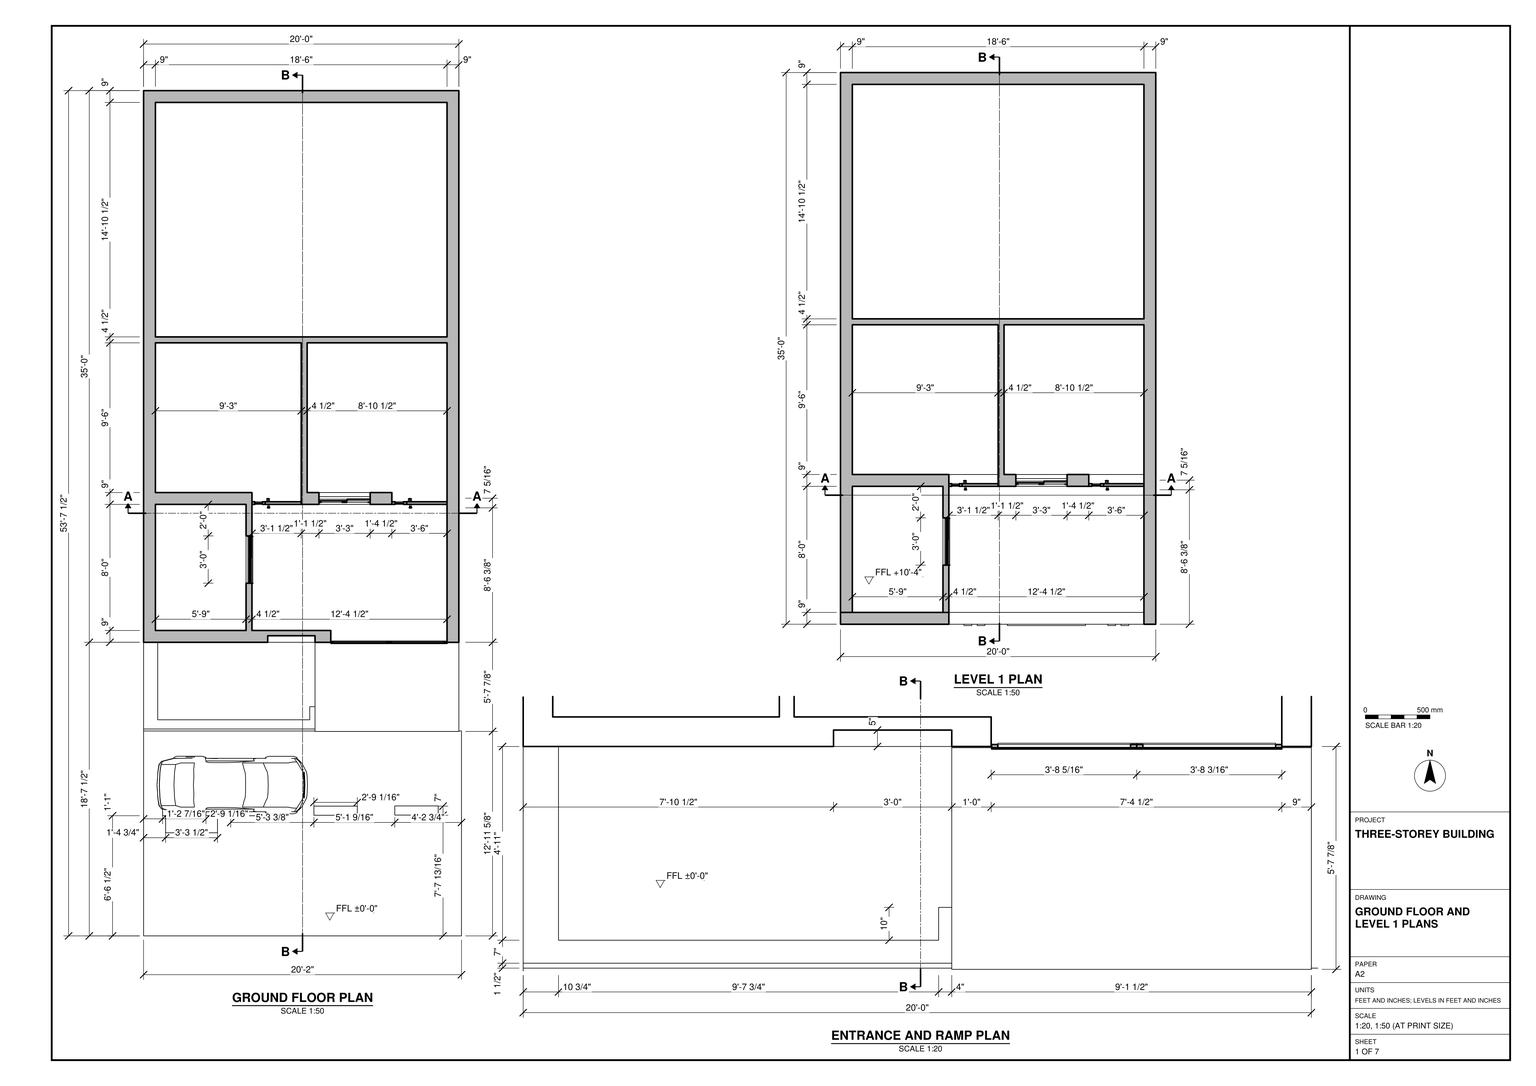
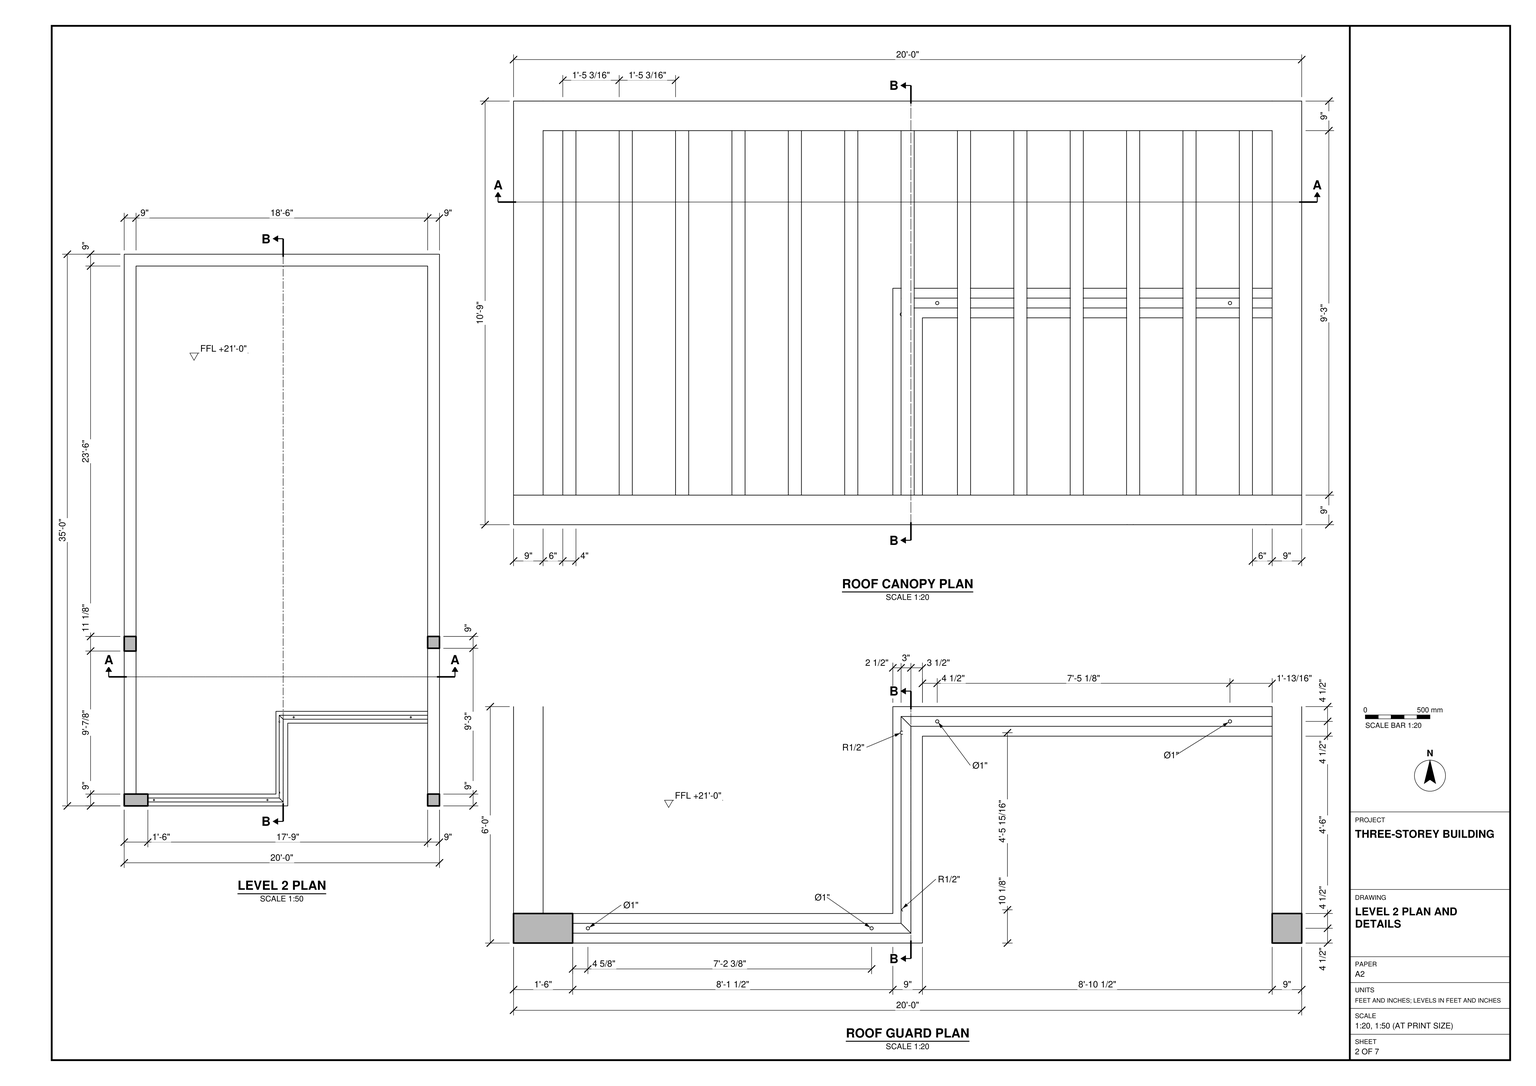
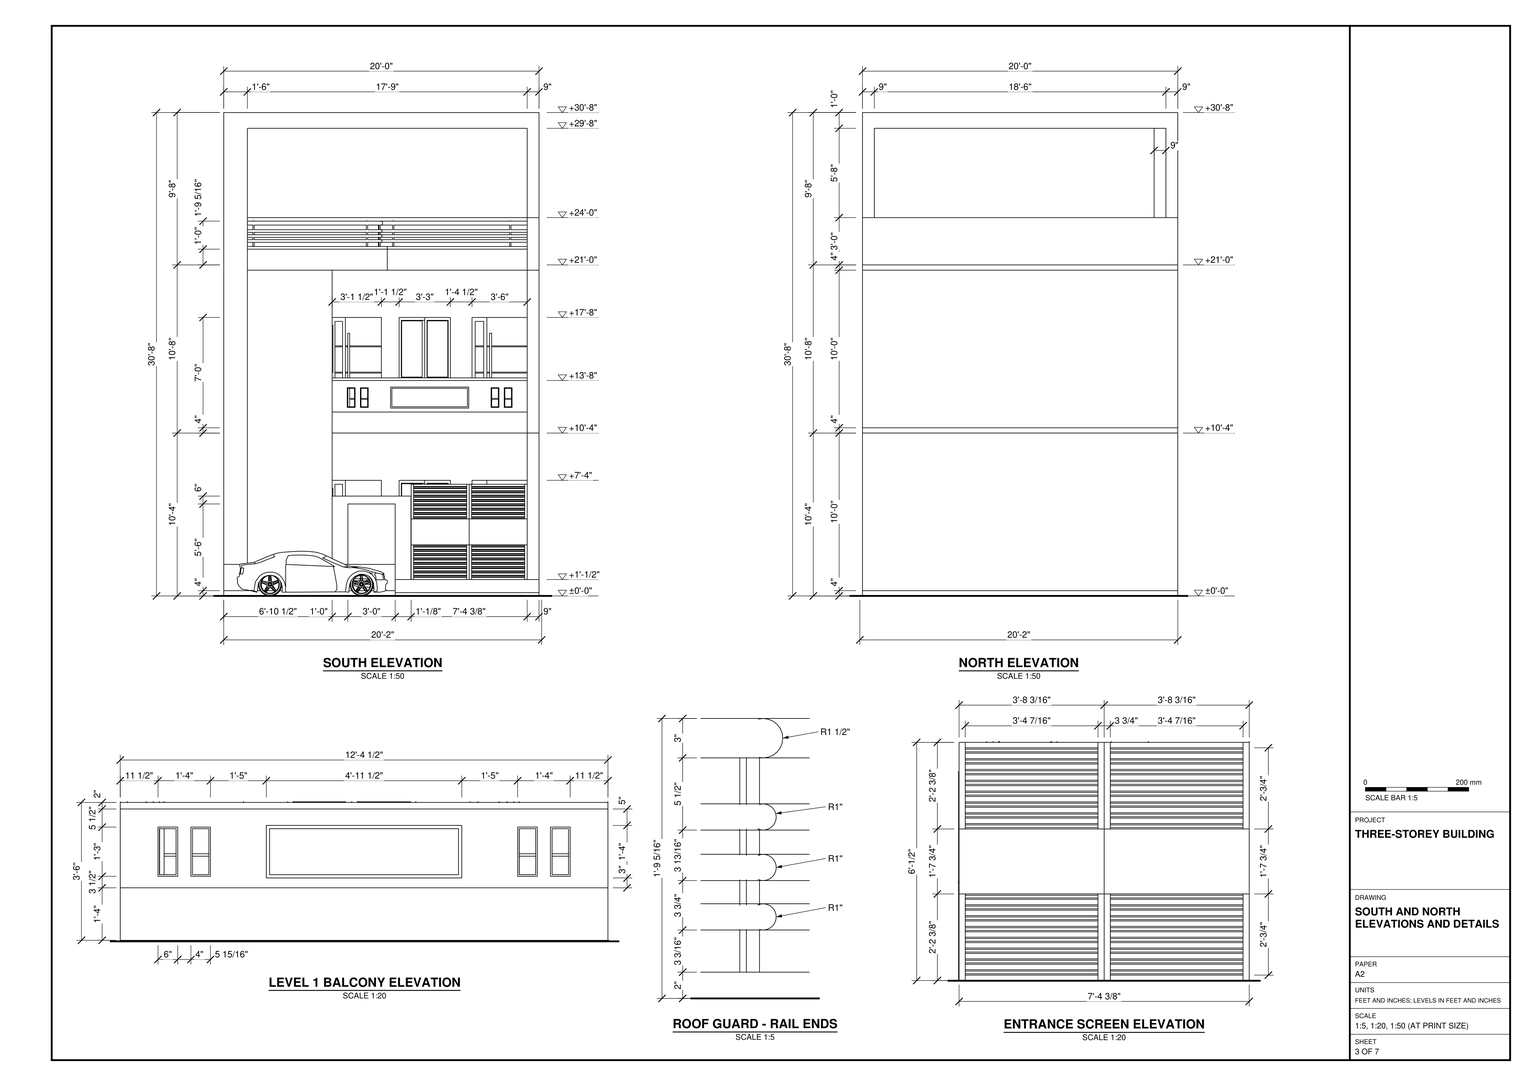
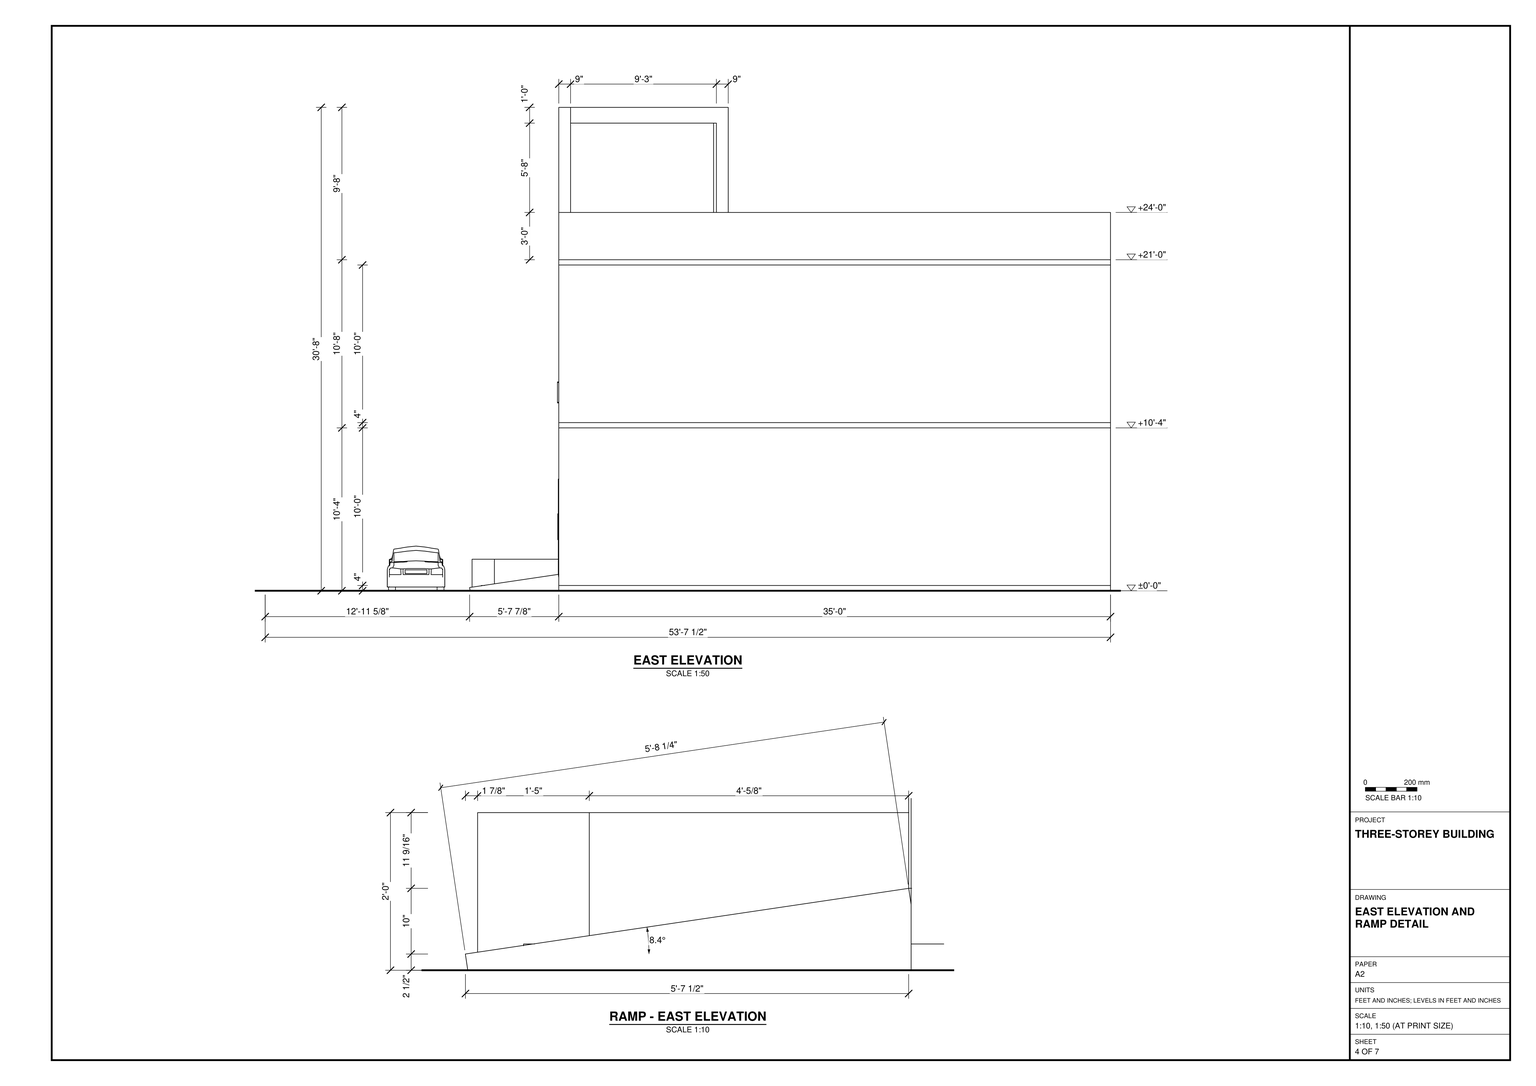
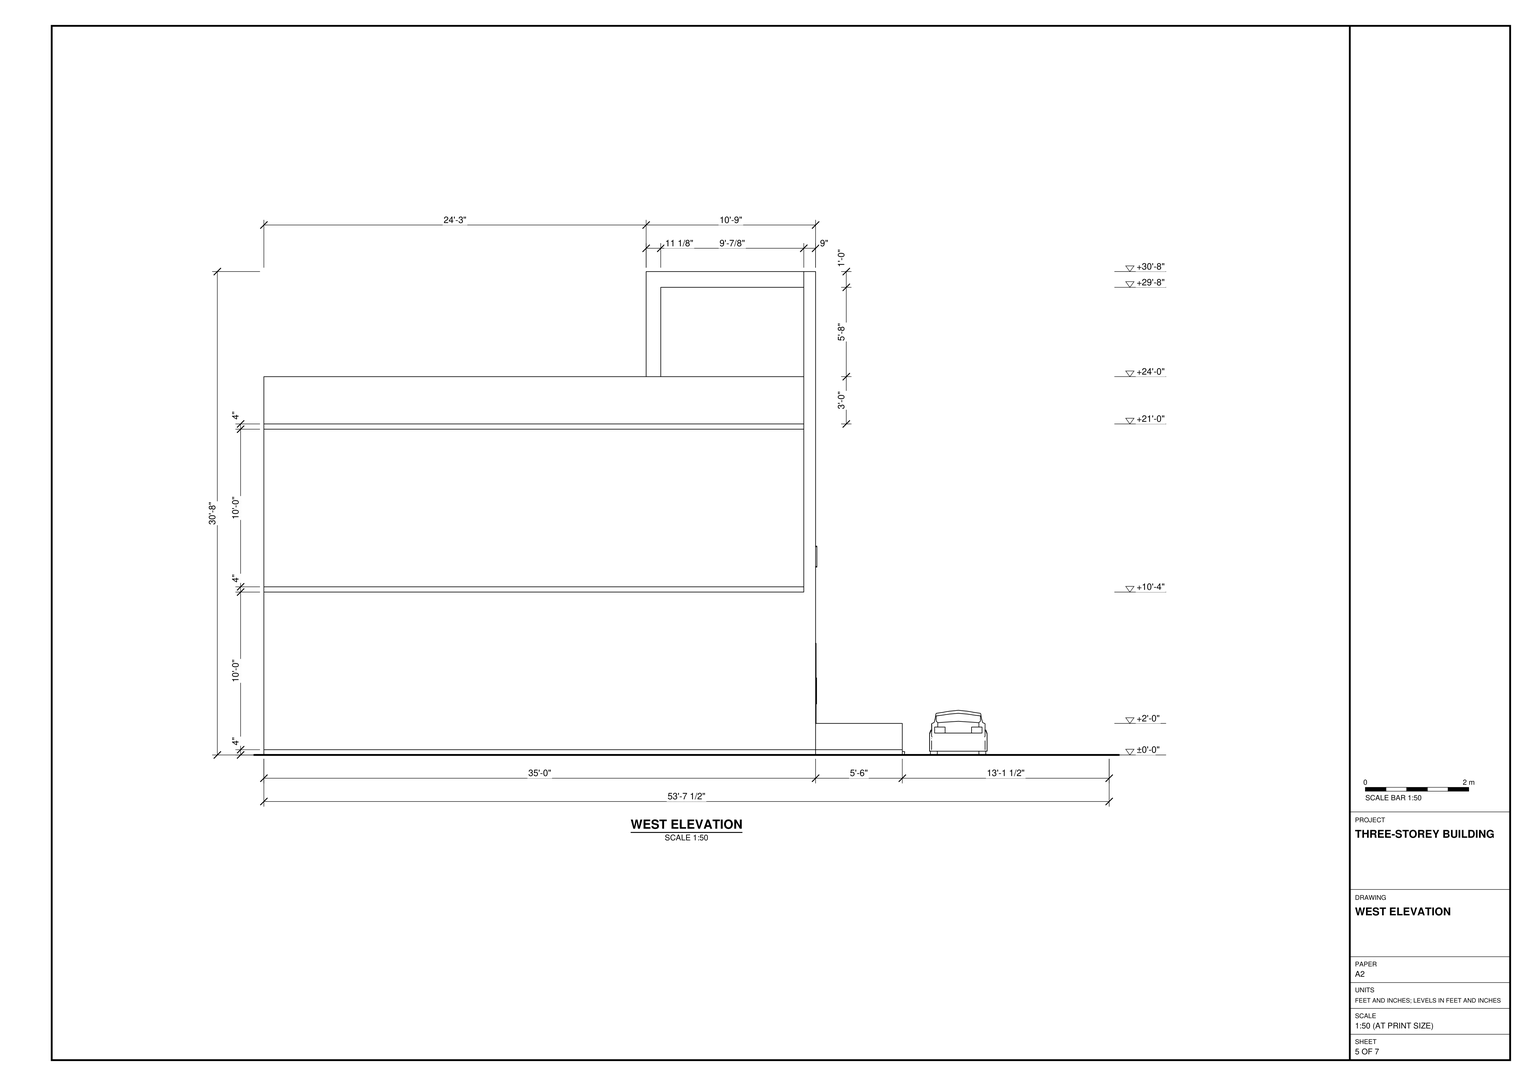
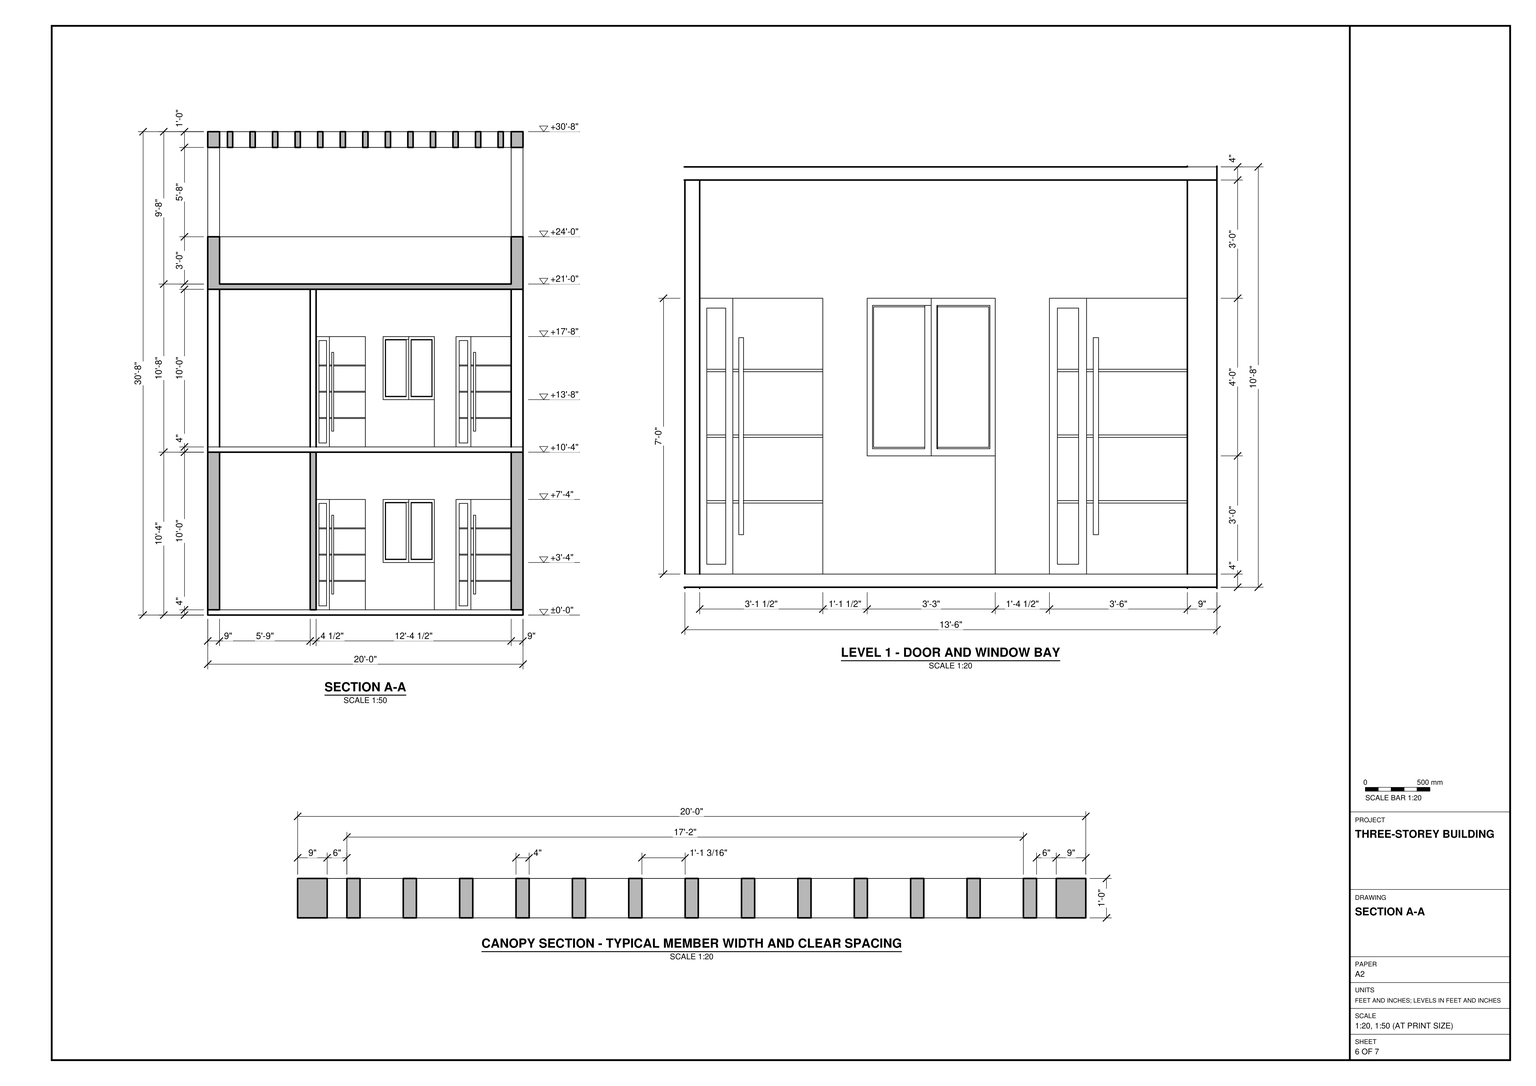
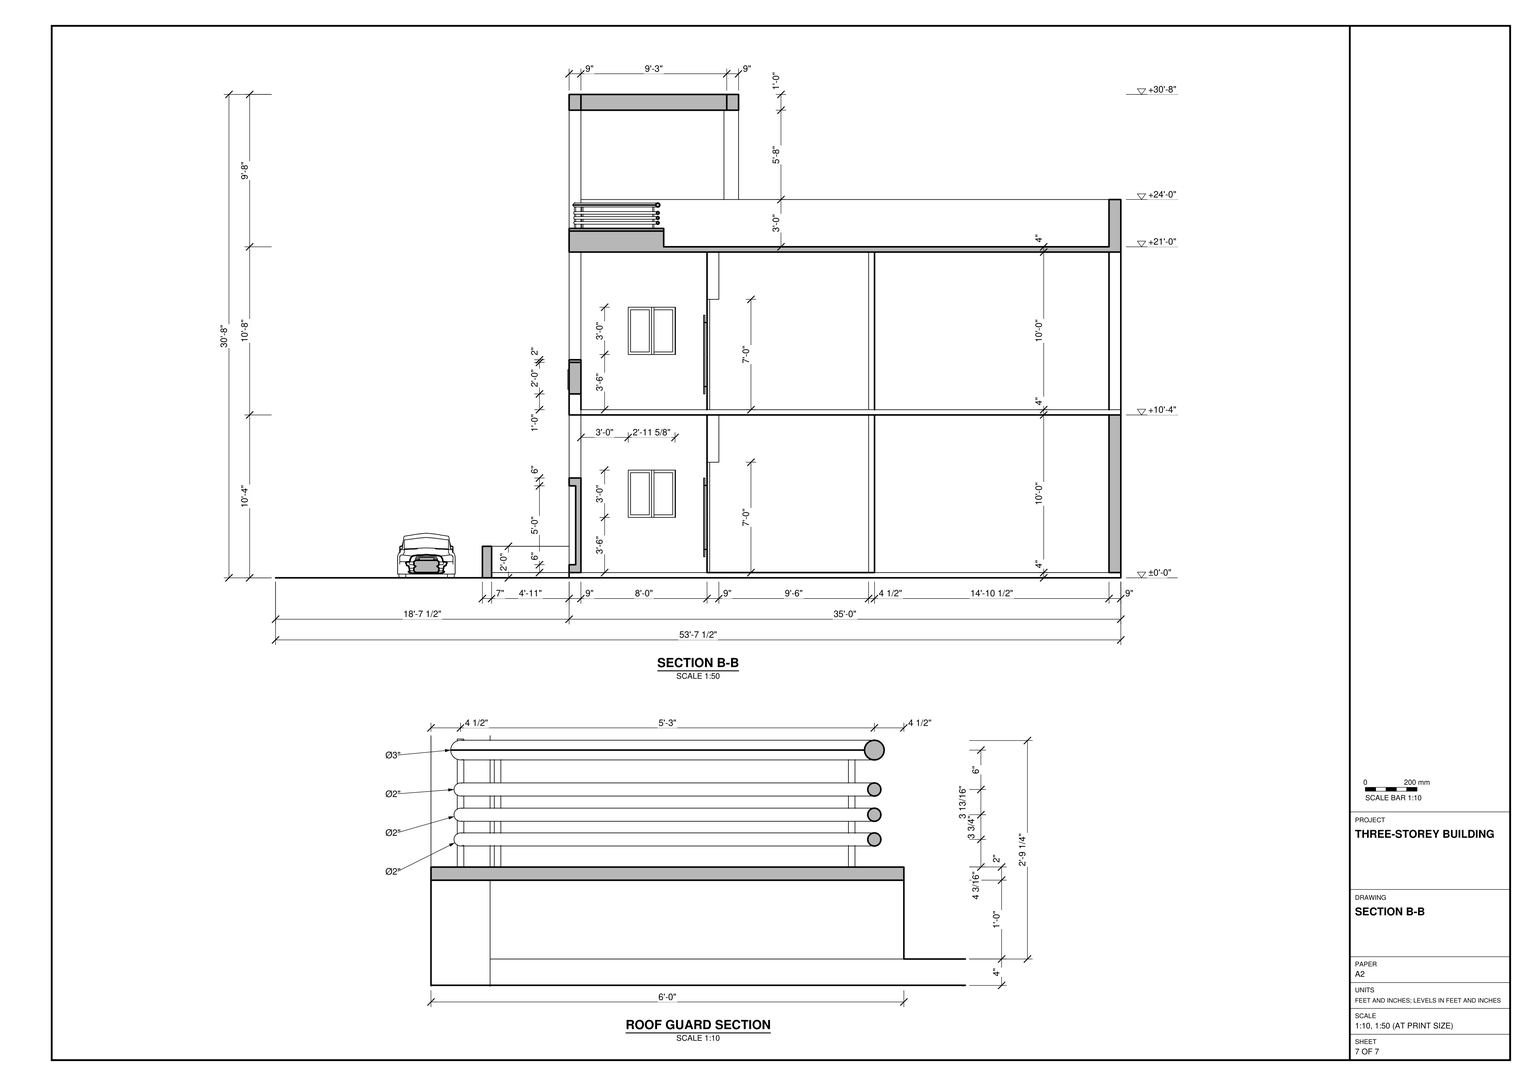
Build the three-storey building and its entrance forecourt in SketchUp from task_files/diagram_01.pdf. Work in feet and inches. The complete model, including the forecourt, is 20'-2" wide, 53'-7 1/2" deep and 30'-8" high. Set the floor levels at ±0'-0", +10'-4" and +21'-0".

Use the 20'-0" by 35'-0" building footprint to lay out the floor slabs and walls. Follow the plans for the 9" perimeter walls, the thinner 4 1/2" partitions and the locations of the door and window openings. On the two lower floors, retain the full-width rear room, the two rooms side by side in the middle and the narrower enclosed space at the front left.

At the south entrance, model the ramp, landing and two-leaf screen. Place the car across the forecourt as shown. Above the entrance, model the recessed openings and the balcony front with its wide central panel and paired narrow panels. At roof level, follow the stepped front edge of the terrace with horizontal guardrails, and build the supported canopy with its parallel overhead members. Decor and loose items, including the car, may be any suitable library components.

Keep walls, slabs, roof elements and each furniture or joinery piece in separate groups or components, and use components for repeated parts. Save one SketchUp model as output_files/three_storey_building_with_roof_terrace_and_ramp.skp.

# SketchUp Ruby script. Lengths in inches.
U = 1.inch
M = Sketchup.active_model
def pt(a) = Geom::Point3d.new(a.map { |v| v * U })
def face(e, loops, mat)
  f = e.add_face(loops[0].map { |a| pt(a) })
  loops[1..].each { |l| e.add_face(l.map { |a| pt(a) }).erase! }
  f.material = f.back_material = mat if mat
  f
end
# faces: each face lists its corners as indices into pts; further lists are holes
def faces(e, pts, list, mat = nil) = list.each { |f| face(e, (f[0].is_a?(Array) ? f : [f]).map { |l| l.map { |i| pts[i] } }, mat) }
# xy, xz, yz: faces in a plane at the given z, y or x. An outline is a flat list of corners, or four numbers for a rectangle; further outlines are holes
def ring(l) = l.size == 4 ? [[l[0], l[1]], [l[2], l[1]], [l[2], l[3]], [l[0], l[3]]] : l.each_slice(2).to_a
def flat(e, list, mat, &to3) = list.each { |f| face(e, (f[0].is_a?(Array) ? f : [f]).map { |l| ring(l).map { |u, v| to3.(u, v) } }, mat) }
def xy(e, z, list, mat = nil) = flat(e, list, mat) { |x, y| [x, y, z] }
def xz(e, y, list, mat = nil) = flat(e, list, mat) { |x, z| [x, y, z] }
def yz(e, x, list, mat = nil) = flat(e, list, mat) { |y, z| [x, y, z] }
def lines(e, pts, list) = list.each { |a, b| e.add_line(pt(pts[a]), pt(pts[b])) }
# prism: a flat outline (further loops are holes) pulled along v
def prism(e, loops, v, mat = nil)
  f = face(e, loops, mat); d = Geom::Vector3d.new(v.map { |x| x * U })
  f.pushpull(f.normal.samedirection?(d) ? d.length : -d.length)
end
def box(e, o, s, mat = nil) = prism(e, [[o, [o[0] + s[0], o[1], o[2]], [o[0] + s[0], o[1] + s[1], o[2]], [o[0], o[1] + s[1], o[2]]]], [0, 0, s[2]], mat)
def at(x, y, z, deg = 0) = Geom::Transformation.translation(pt([x, y, z])) * Geom::Transformation.rotation(ORIGIN, Z_AXIS, deg.degrees)
def axes(o, x, y, z) = Geom::Transformation.new([*x, 0, *y, 0, *z, 0, *pt(o).to_a, 1])
def part(name) = M.definitions.add(name)
# library, detail: a bought-in or finely detailed component or shape, given as its bounding box
def library(name, o, s) = part(name).tap { |d| box(d.entities, o, s) }
def detail(e, o, s) = box(e.add_group.entities, o, s)
def put(e, d, t, mat = nil) = e.add_instance(d, t).tap { |i| i.material = mat if mat }
def group(e, t, mat = nil) = e.add_group.tap { |g| g.transformation = t; g.material = mat if mat }.entities
root = M.entities
M.materials.add("Color_008").color = [30, 30, 30]
M.materials.add("[0055_LightGoldenrodYellow]").color = [250, 250, 210]
M.materials.add("[0131_Silver]").color = [192, 192, 192]
M.materials.add("[0134_DimGray]").color = [105, 105, 105]
M.materials.add("[Color A01]").color = [191, 147, 119]
M.materials.add("[Color C01]").color = [191, 147, 119]
M.materials.add("[Color E03]").color = [255, 255, 104]
M.materials.add("[Color M00]").color = [255, 255, 255]
M.materials.add("[Color M09]").color = [0, 0, 0]
M.materials.add("[Concrete Tile]").color = [203, 190, 164]
M.materials.add("[Field Square Tile]").color = [217, 201, 169]
M.materials.add("[Roofing Slate Tan]").color = [200, 175, 128]
M.materials.add("[Tile Limestone Large]").color = [238, 251, 230]
M.materials.add("[Translucent Glass Blue]").color = [100, 149, 237]
c1 = library("Untitled",[-28.23,109.14,0],[52,7.35,84])
c2 = part("Janela aluminio")
xy(c2.entities,0,[[0,0,47.24,1.57],[23.62,1.57,47.24,2.76],[0,2.76,25.98,3.9375],[0,3.9375,47.24,5.91]])
xy(c2.entities,43.31,[[0,0,47.24,1.57],[23.62,1.57,47.24,2.76],[0,2.76,0,5.91,47.24,5.91,47.24,3.9375,25.98,3.9375,25.98,2.76],[25.98,2.76,47.24,3.9375]])
xz(c2.entities,1.57,[[0,0,23.62,0,23.62,41.34,21.26,41.34,21.26,1.97,1.97,1.97,1.97,41.34,23.62,41.34,23.62,43.31,0,43.31],[[23.62,0,47.24,43.31],[25.7,1.97,45.28,41.34]]])
xz(c2.entities,2.76,[[[0,0,23.62,43.31],[2.36,2.36,21.26,40.94]],[23.62,0,25.98,43.31]])
xz(c2.entities,2.76,[[2.36,2.36,21.26,40.94]],"[Translucent Glass Blue]")
xz(c2.entities,3.9375,[[25.98,0,25.98,2.36,44.88,2.36,44.88,40.94,25.98,40.94,25.98,43.31,47.24,43.31,47.24,0]])
xz(c2.entities,3.9375,[[25.98,2.36,44.88,40.94]],"[Translucent Glass Blue]")
yz(c2.entities,0,[[0,0,1.57,43.31],[2.76,0,5.91,43.31]])
yz(c2.entities,23.62,[[1.57,0,2.76,43.31]])
yz(c2.entities,25.98,[[2.76,0,3.9375,43.31]])
yz(c2.entities,47.24,[[0,0,1.57,43.31],[1.57,0,2.76,43.31],[3.9375,0,5.91,43.31]])
c3 = library("Passenger car",[0,0,0],[114.57,43.85,34.01])
c4 = library("Group\#25",[0,0,0],[240,420,40])
c5 = part("Gate slat")
box(c5.entities,[0,0,-2.03],[1.97,0.97,40.94])
c6 = part("Gate frame member")
box(c6.entities,[0,0,0],[1.9,0.97,93.54])
c7 = part("Gate slat \#1")
box(c7.entities,[2.95,0,-2.03],[0.99,0.97,40.94])
c8 = part("Slatted gate")
p = [[42.85,0.97,43.31],[42.85,0.97,44.29]]
lines(c8.entities,p,[[0,1]])
put(c8.entities,c5,axes([3.9375,0,86.61],[0,0,-1],[0,1,0],[1,0,0]),"Color_008")
put(c8.entities,c6,axes([87.6,0,0],[1,0,0],[0,1,0],[0,0,0.92593]),"Color_008")
put(c8.entities,c5,axes([48.6875,0,86.61],[0,0,-1],[0,1,0],[1,0,0]),"Color_008")
put(c8.entities,c6,axes([0,0,0],[1,0,0],[0,1,0],[0,0,0.92593]),"Color_008")
put(c8.entities,c6,axes([42.85,0,0],[1,0,0],[0,1,0],[0,0,0.92593]),"Color_008")
put(c8.entities,c6,axes([44.75,0,0],[1,0,0],[0,1,0],[0,0,0.92593]),"Color_008")
put(c8.entities,c7,axes([3.9375,0,87.11],[0,0,-1],[0,1,0],[1,0,0]),"[0134_DimGray]")
put(c8.entities,c7,axes([48.6875,0,87.11],[0,0,-1],[0,1,0],[1,0,0]),"[0134_DimGray]")
put(c8.entities,c5,axes([48.6875,0,82.68],[0,0,-1],[0,1,0],[1,0,0]),"Color_008")
put(c8.entities,c7,axes([48.6875,0,83.17],[0,0,-1],[0,1,0],[1,0,0]),"[0134_DimGray]")
put(c8.entities,c7,axes([3.9375,0,83.17],[0,0,-1],[0,1,0],[1,0,0]),"[0134_DimGray]")
put(c8.entities,c5,axes([3.9375,0,82.68],[0,0,-1],[0,1,0],[1,0,0]),"Color_008")
put(c8.entities,c7,axes([48.6875,0,75.3],[0,0,-1],[0,1,0],[1,0,0]),"[0134_DimGray]")
put(c8.entities,c5,axes([48.6875,0,78.74],[0,0,-1],[0,1,0],[1,0,0]),"Color_008")
put(c8.entities,c5,axes([48.6875,0,74.8],[0,0,-1],[0,1,0],[1,0,0]),"Color_008")
put(c8.entities,c7,axes([48.6875,0,79.23],[0,0,-1],[0,1,0],[1,0,0]),"[0134_DimGray]")
put(c8.entities,c7,axes([3.9375,0,75.3],[0,0,-1],[0,1,0],[1,0,0]),"[0134_DimGray]")
put(c8.entities,c5,axes([3.9375,0,78.74],[0,0,-1],[0,1,0],[1,0,0]),"Color_008")
put(c8.entities,c7,axes([3.9375,0,79.23],[0,0,-1],[0,1,0],[1,0,0]),"[0134_DimGray]")
put(c8.entities,c5,axes([3.9375,0,74.8],[0,0,-1],[0,1,0],[1,0,0]),"Color_008")
put(c8.entities,c7,axes([48.6875,0,67.42],[0,0,-1],[0,1,0],[1,0,0]),"[0134_DimGray]")
put(c8.entities,c7,axes([3.9375,0,63.48],[0,0,-1],[0,1,0],[1,0,0]),"[0134_DimGray]")
put(c8.entities,c7,axes([48.6875,0,71.36],[0,0,-1],[0,1,0],[1,0,0]),"[0134_DimGray]")
put(c8.entities,c7,axes([3.9375,0,67.42],[0,0,-1],[0,1,0],[1,0,0]),"[0134_DimGray]")
put(c8.entities,c5,axes([3.9375,0,70.87],[0,0,-1],[0,1,0],[1,0,0]),"Color_008")
put(c8.entities,c5,axes([48.6875,0,70.87],[0,0,-1],[0,1,0],[1,0,0]),"Color_008")
put(c8.entities,c5,axes([48.6875,0,66.93],[0,0,-1],[0,1,0],[1,0,0]),"Color_008")
put(c8.entities,c5,axes([48.6875,0,59.06],[0,0,-1],[0,1,0],[1,0,0]),"Color_008")
put(c8.entities,c5,axes([3.9375,0,55.12],[0,0,-1],[0,1,0],[1,0,0]),"Color_008")
put(c8.entities,c5,axes([3.9375,0,62.99],[0,0,-1],[0,1,0],[1,0,0]),"Color_008")
put(c8.entities,c7,axes([3.9375,0,59.55],[0,0,-1],[0,1,0],[1,0,0]),"[0134_DimGray]")
put(c8.entities,c5,axes([3.9375,0,66.93],[0,0,-1],[0,1,0],[1,0,0]),"Color_008")
put(c8.entities,c5,axes([48.6875,0,62.99],[0,0,-1],[0,1,0],[1,0,0]),"Color_008")
put(c8.entities,c7,axes([48.6875,0,59.55],[0,0,-1],[0,1,0],[1,0,0]),"[0134_DimGray]")
put(c8.entities,c7,axes([48.6875,0,63.48],[0,0,-1],[0,1,0],[1,0,0]),"[0134_DimGray]")
put(c8.entities,c5,axes([3.9375,0,59.06],[0,0,-1],[0,1,0],[1,0,0]),"Color_008")
put(c8.entities,c7,axes([3.9375,0,71.36],[0,0,-1],[0,1,0],[1,0,0]),"[0134_DimGray]")
put(c8.entities,c7,axes([3.9375,0,33.96],[0,0,-1],[0,1,0],[1,0,0]),"[0134_DimGray]")
put(c8.entities,c7,axes([48.6875,0,33.96],[0,0,-1],[0,1,0],[1,0,0]),"[0134_DimGray]")
put(c8.entities,c5,axes([3.9375,0,29.53],[0,0,-1],[0,1,0],[1,0,0]),"Color_008")
put(c8.entities,c7,axes([3.9375,0,26.08],[0,0,-1],[0,1,0],[1,0,0]),"[0134_DimGray]")
put(c8.entities,c5,axes([3.9375,0,33.46],[0,0,-1],[0,1,0],[1,0,0]),"Color_008")
put(c8.entities,c5,axes([48.6875,0,29.53],[0,0,-1],[0,1,0],[1,0,0]),"Color_008")
put(c8.entities,c7,axes([48.6875,0,30.02],[0,0,-1],[0,1,0],[1,0,0]),"[0134_DimGray]")
put(c8.entities,c5,axes([3.9375,0,25.59],[0,0,-1],[0,1,0],[1,0,0]),"Color_008")
put(c8.entities,c5,axes([48.6875,0,25.59],[0,0,-1],[0,1,0],[1,0,0]),"Color_008")
put(c8.entities,c5,axes([48.6875,0,33.46],[0,0,-1],[0,1,0],[1,0,0]),"Color_008")
put(c8.entities,c5,axes([3.9375,0,49.7],[0,0,-1],[0,1,0],[1,0,0]),"Color_008")
put(c8.entities,c7,axes([48.6875,0,26.08],[0,0,-1],[0,1,0],[1,0,0]),"[0134_DimGray]")
put(c8.entities,c7,axes([3.9375,0,30.02],[0,0,-1],[0,1,0],[1,0,0]),"[0134_DimGray]")
put(c8.entities,c5,axes([3.9375,0,5.91],[0,0,-1],[0,1,0],[1,0,0]),"Color_008")
put(c8.entities,c5,axes([48.6875,0,13.78],[0,0,-1],[0,1,0],[1,0,0]),"Color_008")
put(c8.entities,c7,axes([48.6875,0,10.33],[0,0,-1],[0,1,0],[1,0,0]),"[0134_DimGray]")
put(c8.entities,c7,axes([3.9375,0,6.4],[0,0,-1],[0,1,0],[1,0,0]),"[0134_DimGray]")
put(c8.entities,c5,axes([3.9375,0,13.78],[0,0,-1],[0,1,0],[1,0,0]),"Color_008")
put(c8.entities,c5,axes([48.6875,0,21.65],[0,0,-1],[0,1,0],[1,0,0]),"Color_008")
put(c8.entities,c5,axes([48.6875,0,5.91],[0,0,-1],[0,1,0],[1,0,0]),"Color_008")
put(c8.entities,c7,axes([48.6875,0,22.15],[0,0,-1],[0,1,0],[1,0,0]),"[0134_DimGray]")
put(c8.entities,c5,axes([48.6875,0,1.97],[0,0,-1],[0,1,0],[1,0,0]),"Color_008")
put(c8.entities,c5,axes([48.6875,0,9.84],[0,0,-1],[0,1,0],[1,0,0]),"Color_008")
put(c8.entities,c7,axes([48.6875,0,6.4],[0,0,-1],[0,1,0],[1,0,0]),"[0134_DimGray]")
put(c8.entities,c5,axes([3.9375,0,9.84],[0,0,-1],[0,1,0],[1,0,0]),"Color_008")
put(c8.entities,c7,axes([3.9375,0,10.33],[0,0,-1],[0,1,0],[1,0,0]),"[0134_DimGray]")
put(c8.entities,c7,axes([3.9375,0,22.15],[0,0,-1],[0,1,0],[1,0,0]),"[0134_DimGray]")
put(c8.entities,c5,axes([3.9375,0,1.97],[0,0,-1],[0,1,0],[1,0,0]),"Color_008")
put(c8.entities,c7,axes([3.9375,0,18.21],[0,0,-1],[0,1,0],[1,0,0]),"[0134_DimGray]")
put(c8.entities,c7,axes([3.9375,0,14.27],[0,0,-1],[0,1,0],[1,0,0]),"[0134_DimGray]")
put(c8.entities,c5,axes([3.9375,0,21.65],[0,0,-1],[0,1,0],[1,0,0]),"Color_008")
put(c8.entities,c7,axes([48.6875,0,18.21],[0,0,-1],[0,1,0],[1,0,0]),"[0134_DimGray]")
put(c8.entities,c5,axes([3.9375,0,17.72],[0,0,-1],[0,1,0],[1,0,0]),"Color_008")
put(c8.entities,c5,axes([48.6875,0,17.72],[0,0,-1],[0,1,0],[1,0,0]),"Color_008")
put(c8.entities,c7,axes([48.6875,0,14.27],[0,0,-1],[0,1,0],[1,0,0]),"[0134_DimGray]")
put(c8.entities,c5,axes([3.9375,0,44.29],[0,0,-1],[0,1,0],[1,0,0]),"Color_008")
put(c8.entities,c5,axes([3.9375,0,38.88],[0,0,-1],[0,1,0],[1,0,0]),"Color_008")
put(c8.entities,c5,axes([48.6875,0,49.7],[0,0,-1],[0,1,0],[1,0,0]),"Color_008")
put(c8.entities,c5,axes([48.6875,0,44.29],[0,0,-1],[0,1,0],[1,0,0]),"Color_008")
put(c8.entities,c5,axes([48.6875,0,38.88],[0,0,-1],[0,1,0],[1,0,0]),"Color_008")
put(c8.entities,c5,axes([48.6875,0,55.12],[0,0,-1],[0,1,0],[1,0,0]),"Color_008")
c9 = part("Glass panel \#1")
box(c9.entities,[0,0,-1.97],[52.81,0.39,23.62])
c10 = part("Glass panel")
box(c10.entities,[0,0,-9.84],[39.64,0.39,36.58])
xy(root,19.1,[[0,156,130.5,223.5]])
xy(root,19.1,[[66.31,91.44,99.35,98.41],[14.46,91.5,47.5,98.47],[129.67,91.8125,162.71,98.78],[191.22,91.96,224.26,98.93]],"[Color M00]")
xy(root,19.1,[[[0,0,242,156],[16.76,78.5,16.76,91.5,14.46,91.5,14.46,98.47,47.5,98.47,47.5,91.5,56.26,91.5,56.26,78.5],[66.31,91.44,99.35,98.41],[129.67,91.8125,162.71,98.78],[191.22,91.96,224.26,98.93]],[16.76,78.5,56.26,91.5]],"[Color M09]")
xy(root,307.1,[[0,341.375,9,352.5],[231,343.5,240,352.5]])
xy(root,375.1,[[0,232.5,9,341.375],[231,232.5,240,343.5],[9,343.5,231,352.5]])
xy(root,387.1,[[0,232.5,9,232.5,9,343.5,231,343.5,231,232.5,240,232.5,240,352.5,0,352.5]])
xz(root,232.5,[[0,375.1,9,387.1],[231,375.1,240,387.1]])
xz(root,341.375,[[0,307.1,9,375.1]])
xz(root,343.5,[[231,307.1,240,375.1],[9,375.1,15,387.1],[19,375.1,231,387.1]])
xz(root,352.5,[[0,307.1,0,387.1,240,387.1,240,307.1,231,307.1,231,375.1,9,375.1,9,307.1]])
yz(root,0,[[341.375,307.1,341.375,375.1,232.5,375.1,232.5,387.1,352.5,387.1,352.5,307.1]])
yz(root,9,[[341.375,307.1,352.5,307.1,352.5,375.1,343.5,375.1,343.5,387.1,232.5,387.1,232.5,375.1,341.375,375.1]])
yz(root,231,[[343.5,307.1,352.5,375.1],[232.5,375.1,343.5,387.1]])
yz(root,240,[[343.5,307.1,352.5,307.1,352.5,387.1,232.5,387.1,232.5,375.1,343.5,375.1]])
# 4 loose lines left out
put(root,c1,axes([211.8,216.7,23.1],[0.80769,0,0],[0,1,0],[0,0,1]))
put(root,c1,axes([102.86,216.7,23.1],[0.72115,0,0],[0,1,0],[0,0,1]))
put(root,c2,axes([133.5,328.5,59.1],[0.8255,0,0],[0,1,0],[0,0,1.10836]))
put(root,c2,axes([79.41,268.5,65.1],[0,0.75438,0],[0.6325,0,0],[0,0,0.83127]))
put(root,c1,axes([102.86,216.7,147.1],[0.72115,0,0],[0,1,0],[0,0,1]))
put(root,c1,axes([211.8,216.7,147.1],[0.80769,0,0],[0,1,0],[0,0,1]))
put(root,c2,axes([133.5,328.5,183.1],[0.8255,0,0],[0,1,0],[0,0,1.10836]))
put(root,c2,axes([79.41,268.5,189.1],[0,0.75438,0],[0.6325,0,0],[0,0,0.83127]))
put(root,c3,at(124.73,136.77,19.1,-180))
g1 = group(root,at(0,223.5,23.1))
xy(g1,0,[[[0,0,0,420,240,420,240,0,231,0,231,228,124.5,228,124.5,114,172.5,114,172.5,105,120,105,120,228,9,228,9,114,82.5,114,82.5,9,142.5,9,142.5,0],[9,232.5,231,411],[9,9,78,105]],[172.5,105,189,114]],"[Color M00]")
xy(g1,6,[[94.5,0,130.5,5]],"[Color M00]")
xy(g1,36,[[133.5,105,172.5,114]],"[Color M00]")
xy(g1,42,[[78,45,82.5,81]],"[Color M00]")
xy(g1,66,[[94.5,0,130.5,5]],"[Color M00]")
xy(g1,72,[[82.5,0,142.5,9]],"[Color M00]")
xy(g1,78,[[78,45,82.5,81]],"[Color M00]")
xy(g1,84,[[82.5,105,120,114],[133.5,105,172.5,114],[189,105,231,114]],"[Color M00]")
xy(g1,120,[[[231,0,240,0,240,420,0,420,0,9,9,9,9,105,78,105,78,9,82.5,9,82.5,105,231,105,231,114,124.5,114,124.5,228,231,228],[9,232.5,231,411],[9,114,120,228]],[9,9,78,105]],"[Color M00]")
xy(g1,244,[[18,0,82.5,9]],"[Color M00]")
xy(g1,284,[[231,0,240,9]],"[Color M00]")
xy(g1,352,[[18,0,231,9]],"[Color M00]")
xy(g1,364,[[0,0,240,9]],"[Color M00]")
xz(g1,0,[[18,0,82.5,244]],"[Color C01]")
xz(g1,0,[[0,0,18,0,18,352,231,352,231,284,240,284,240,364,0,364],[[82.5,0,142.5,72],[94.5,6,130.5,66]],[231,0,240,120]],"[Color M00]")
xz(g1,5,[[94.5,6,130.5,66]],"[Color A01]")
xz(g1,9,[[9,0,78,120],[82.5,0,142.5,72],[0,120,0,352,18,352,18,244,78,244,78,120],[78,120,82.5,244],[231,284,231,352,0,352,0,364,240,364,240,284]],"[Color M00]")
xz(g1,45,[[78,42,82.5,78]],"[Color M00]")
xz(g1,81,[[78,42,82.5,78]],"[Color M00]")
xz(g1,105,[[9,0,78,120],[120,0,172.5,0,172.5,36,133.5,36,133.5,84,172.5,84,172.5,0,189,0,189,84,231,84,231,120,82.5,120,82.5,84,120,84]],"[Color M00]")
xz(g1,114,[[9,0,9,120,120,120,120,84,82.5,84,82.5,0],[[124.5,0,124.5,120,231,120,231,84,189,84,189,0],[133.5,36,172.5,84]]],"[Color M00]")
xz(g1,228,[[9,0,120,120],[124.5,0,231,120]],"[Color M00]")
xz(g1,232.5,[[9,0,231,120]],"[Color M00]")
xz(g1,411,[[9,0,231,120]],"[Color M00]")
xz(g1,420,[[0,0,240,120]],"[Color M00]")
yz(g1,0,[[0,0,0,364,9,364,9,120,420,120,420,0]],"[Color M00]")
yz(g1,9,[[9,0,105,120],[114,0,228,120],[232.5,0,411,120]],"[Color M00]")
yz(g1,18,[[0,244,9,352]],"[Color M00]")
yz(g1,78,[[9,0,9,120,81,120,81,78,45,78,45,42,81,42,81,0],[81,0,105,120]],"[Color M00]")
yz(g1,82.5,[[[9,0,114,0,114,84,105,84,105,120,9,120],[45,42,81,78]],[0,72,9,244]],"[Color M00]")
yz(g1,94.5,[[0,6,5,66]],"[Color M00]")
yz(g1,120,[[105,0,105,84,114,84,114,120,228,120,228,0]],"[Color M00]")
yz(g1,124.5,[[114,0,228,120]],"[Color M00]")
yz(g1,130.5,[[0,6,5,66]],"[Color M00]")
yz(g1,133.5,[[105,36,114,84]],"[Color M00]")
yz(g1,142.5,[[0,0,9,72]],"[Color M00]")
yz(g1,172.5,[[105,36,114,84]],"[Color M00]")
yz(g1,189,[[105,0,114,84]],"[Color M00]")
yz(g1,231,[[0,0,0,120,105,120,105,84,114,84,114,120,228,120,228,0],[232.5,0,411,120],[0,284,9,352]],"[Color M00]")
yz(g1,240,[[0,0,420,120],[0,284,9,364]],"[Color M00]")
g2 = group(root,at(0,223.5,23.1),"[Field Square Tile]")
xy(g2,-4,[[130.5,-67.5,240,0],[0,-66,0,0,10.75,0,10.75,-59,130.5,-59,130.5,-66],[0,0,240,420]])
xy(g2,0,[[126.5,-59,130.5,-49]])
xy(g2,20,[[0,-66,130.5,-66,130.5,-49,126.5,-49,126.5,-59,10.75,-59,10.75,0,0,0]],"[Concrete Tile]")
xz(g2,-66,[[0,-4,130.5,0],[0,0,130.5,20]],"[Concrete Tile]")
xz(g2,-59,[[10.75,-4,130.5,0],[10.75,0,126.5,20]])
xz(g2,-49,[[126.5,0,130.5,20]])
xz(g2,0,[[0,-4,10.75,0],[10.75,-4,130.5,0],[130.5,-4,240,6],[0,0,10.75,20]])
xz(g2,420,[[0,-4,240,0]])
yz(g2,0,[[-66,-4,0,0],[0,-4,420,0]])
yz(g2,0,[[-66,0,0,20]],"[Concrete Tile]")
yz(g2,10.75,[[-59,-4,0,0],[-59,0,0,20]])
yz(g2,126.5,[[-59,0,-49,20]])
yz(g2,130.5,[[-67.5,-4,-67.87,-1.53,-66,-1.25,-66,-4],[-66,-4,-59,-4,-59,-0.21,-66,-1.25],[-66,-1.25,-59,-0.21,-59,0,-57.56,0,-49,1.27,-49,20,-66,20],[-57.56,0,-49,1.27,-49,0]])
yz(g2,130.5,[[-59,-4,-59,-0.21,-57.56,0,-49,0,-49,1.27,-0.37,8.47,0,6,0,-4]],"[Roofing Slate Tan]")
yz(g2,240,[[-67.5,-4,0,-4,0,6,-0.37,8.47,-67.87,-1.53],[0,-4,420,0]])
p = [[130.5,-67.5,-4],[240,-67.5,-4],[240,-67.87,-1.53],[130.5,-67.87,-1.53],[130.5,-0.37,8.47],[130.5,-49,1.27],
  [130.5,-57.56,0],[130.5,-59,-0.21],[130.5,-66,-1.25],[240,-0.37,8.47],[240,0,6],[130.5,0,6]]
faces(g2,p,[[0,1,2,3],[4,5,6,7,8,3,2,9]],"[Roofing Slate Tan]")
faces(g2,p,[[10,11,4,9]])
g3 = group(root,at(0,223.5,147.1))
xy(g3,0,[[172.5,105,189,114]])
xy(g3,36,[[133.5,105,172.5,114]])
xy(g3,42,[[78,45,82.5,81]])
xy(g3,78,[[78,45,82.5,81]])
xy(g3,84,[[82.5,105,120,114],[133.5,105,172.5,114],[189,105,231,114]])
xy(g3,120,[[[231,0,240,0,240,420,0,420,0,9,9,9,9,105,78,105,78,9,82.5,9,82.5,105,231,105,231,114,124.5,114,124.5,228,231,228],[9,232.5,231,411],[9,114,120,228]]])
xz(g3,0,[[231,-4,240,120]])
xz(g3,9,[[0,0,9,120],[9,0,78,120],[78,0,82.5,120]])
xz(g3,45,[[78,42,82.5,78]])
xz(g3,81,[[78,42,82.5,78]])
xz(g3,105,[[9,0,78,120]])
xz(g3,105,[[120,0,172.5,0,172.5,36,133.5,36,133.5,84,172.5,84,172.5,0,189,0,189,84,231,84,231,120,82.5,120,82.5,84,120,84]],"[Tile Limestone Large]")
xz(g3,114,[[9,0,9,120,120,120,120,84,82.5,84,82.5,0],[[124.5,0,124.5,120,231,120,231,84,189,84,189,0],[133.5,36,172.5,84]]])
xz(g3,228,[[9,0,120,120],[124.5,0,231,120]])
xz(g3,232.5,[[9,0,231,120]])
xz(g3,411,[[9,0,231,120]])
xz(g3,420,[[0,0,240,120]])
yz(g3,0,[[9,0,420,120]],"[Color M00]")
yz(g3,9,[[9,0,105,120],[114,0,228,120],[232.5,0,411,120]])
yz(g3,78,[[9,0,9,120,81,120,81,78,45,78,45,42,81,42,81,0],[81,0,105,120]])
yz(g3,82.5,[[[9,0,114,0,114,84,105,84,105,120,9,120],[45,42,81,78]]],"[Tile Limestone Large]")
yz(g3,120,[[105,0,105,84,114,84,114,120,228,120,228,0]])
yz(g3,124.5,[[114,0,228,120]])
yz(g3,133.5,[[105,36,114,84]])
yz(g3,172.5,[[105,36,114,84]])
yz(g3,189,[[105,0,114,84]])
yz(g3,231,[[232.5,0,411,120]])
yz(g3,231,[[0,0,0,120,105,120,105,84,114,84,114,120,228,120,228,0]],"[Tile Limestone Large]")
yz(g3,240,[[0,0,420,120]],"[Color M00]")
g4 = group(root,at(0,223.5,147.1))
xy(g4,-4,[[82.5,0,82.5,9,0,9,0,420,240,420,240,0]])
xy(g4,12,[[82.5,0,231,9]])
xy(g4,15,[[126.98,-1,186.5,0]])
xy(g4,15.5,[[94,-1,100,0],[203.5,-1,209.5,0],[213.5,-1,219.5,0]])
xy(g4,15.52,[[104.02,-1,109.98,0]])
xy(g4,16,[[94.5,-1,99.5,9],[104.5,-1,109.5,9],[127.98,-1,185.5,4],[204,-1,209,9],[214,-1,219,9]])
xy(g4,30,[[94.5,-1,99.5,9],[104.5,-1,109.5,9],[127.98,-1,185.5,4],[204,-1,209,9],[214,-1,219,9]])
xy(g4,30.48,[[104.02,-1,109.98,0]],"[Color E03]")
xy(g4,30.5,[[94,-1,100,0],[203.5,-1,209.5,0],[213.5,-1,219.5,0]],"[Color E03]")
xy(g4,31,[[126.98,-1,186.5,0]],"[Color E03]")
xy(g4,36,[[82.5,0,231,9]])
xy(g4,38,[[82.5,0,231,9]])
xz(g4,-1,[[[126.98,15,186.5,31],[127.98,16,185.5,30]],[[94,15.5,100,30.5],[94.5,16,99.5,30]],[[203.5,15.5,209.5,30.5],[204,16,209,30]],[[213.5,15.5,219.5,30.5],[214,16,219,30]],[[104.02,15.52,109.98,30.48],[104.5,16,109.5,30]]],"[Color E03]")
xz(g4,0,[[[82.5,12,231,36],[126.98,15,186.5,31],[94,15.5,100,30.5],[203.5,15.5,209.5,30.5],[213.5,15.5,219.5,30.5],[104.02,15.52,109.98,30.48]],[82.5,36,231,38]])
xz(g4,0,[[82.5,-4,231,12]],"[Color E03]")
xz(g4,4,[[127.98,16,185.5,30]],"[Translucent Glass Blue]")
xz(g4,9,[[0,-4,82.5,0],[82.5,0,231,12],[[82.5,12,231,36],[94.5,16,99.5,30],[104.5,16,109.5,30],[204,16,209,30],[214,16,219,30]],[82.5,36,231,38]])
xz(g4,420,[[0,-4,240,0]])
yz(g4,0,[[9,-4,420,0]])
yz(g4,82.5,[[0,-4,9,12],[0,12,9,36],[0,36,9,38]])
yz(g4,94,[[-1,15.5,0,30.5]],"[Color E03]")
yz(g4,94.5,[[-1,16,9,30]])
yz(g4,99.5,[[-1,16,9,30]])
yz(g4,100,[[-1,15.5,0,30.5]])
yz(g4,104.02,[[-1,15.52,0,30.48]],"[Color E03]")
yz(g4,104.5,[[-1,16,9,30]])
yz(g4,109.5,[[-1,16,9,30]])
yz(g4,109.98,[[-1,15.52,0,30.48]],"[Color E03]")
yz(g4,126.98,[[-1,15,0,31]],"[Color E03]")
yz(g4,127.98,[[-1,16,4,30]])
yz(g4,185.5,[[-1,16,4,30]])
yz(g4,186.5,[[-1,15,0,31]],"[Color E03]")
yz(g4,203.5,[[-1,15.5,0,30.5]],"[Color E03]")
yz(g4,204,[[-1,16,9,30]])
yz(g4,209,[[-1,16,9,30]])
yz(g4,209.5,[[-1,15.5,0,30.5]],"[Color E03]")
yz(g4,213.5,[[-1,15.5,0,30.5]],"[Color E03]")
yz(g4,214,[[-1,16,9,30]])
yz(g4,219,[[-1,16,9,30]])
yz(g4,219.5,[[-1,15.5,0,30.5]],"[Color E03]")
yz(g4,231,[[0,0,9,12],[0,12,9,36],[0,36,9,38]])
yz(g4,240,[[0,-4,420,0]])
g5 = group(root,at(15,343.5,375.1))
box(g5,[0,-111,0],[4,111,12])
g6 = group(root,at(32.17,343.5,375.1))
box(g6,[0,-111,0],[4,111,12])
g7 = group(root,at(49.33,343.5,375.1))
box(g7,[0,-111,0],[4,111,12])
g8 = group(root,at(66.5,343.5,375.1))
box(g8,[0,-111,0],[4,111,12])
g9 = group(root,at(83.67,343.5,375.1))
box(g9,[0,-111,0],[4,111,12])
g10 = group(root,at(100.83,343.5,375.1))
box(g10,[0,-111,0],[4,111,12])
g11 = group(root,at(118,343.5,375.1))
box(g11,[0,-111,0],[4,111,12])
g12 = group(root,at(135.17,343.5,375.1))
box(g12,[0,-111,0],[4,111,12])
g13 = group(root,at(152.33,343.5,375.1))
box(g13,[0,-111,0],[4,111,12])
g14 = group(root,at(169.5,343.5,375.1))
box(g14,[0,-111,0],[4,111,12])
g15 = group(root,at(186.67,343.5,375.1))
box(g15,[0,-111,0],[4,111,12])
g16 = group(root,at(203.83,343.5,375.1))
box(g16,[0,-111,0],[4,111,12])
g17 = group(root,at(221,343.5,375.1))
box(g17,[0,-111,0],[4,111,12])
put(root,c4,at(0,223.5,267.1))
g18 = group(root,at(142.65,222.74,31.58))
put(g18,c8,axes([0,0.39,0],[0.9871,0,0],[0,1,0],[0,0,0.83731]),"[0055_LightGoldenrodYellow]")
put(g18,c9,axes([0,0,28.02],[0.83651,0,0],[0,1,0],[0,0,0.83731]),"Color_008")
put(g18,c10,axes([44.17,1.36,52.8],[1.0671,0,0],[0,1,0],[0,0,0.67588]),"[0131_Silver]")
put(g18,c10,axes([1.88,1.36,8.3],[1.0671,0,0],[0,1,0],[0,0,0.67588]),"[0131_Silver]")
put(g18,c10,axes([1.88,1.36,52.8],[1.0671,0,0],[0,1,0],[0,0,0.67588]),"[0131_Silver]")
put(g18,c9,axes([44.17,0,28.02],[0.83651,0,0],[0,1,0],[0,0,0.83731]),"Color_008")
put(g18,c10,axes([44.17,1.36,8.3],[1.0671,0,0],[0,1,0],[0,0,0.67588]),"[0131_Silver]")
